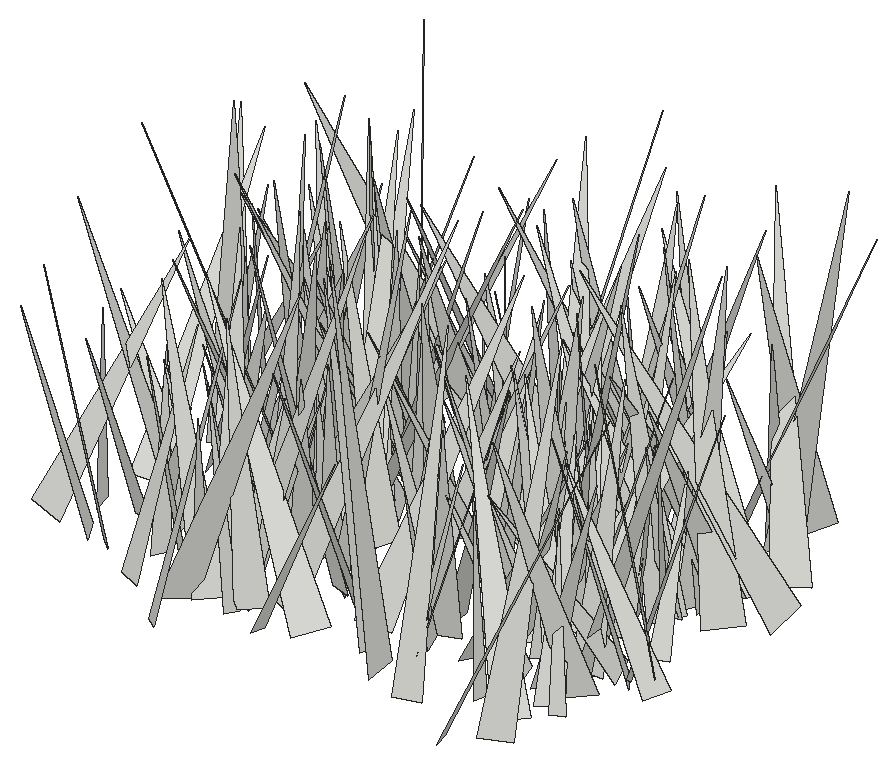
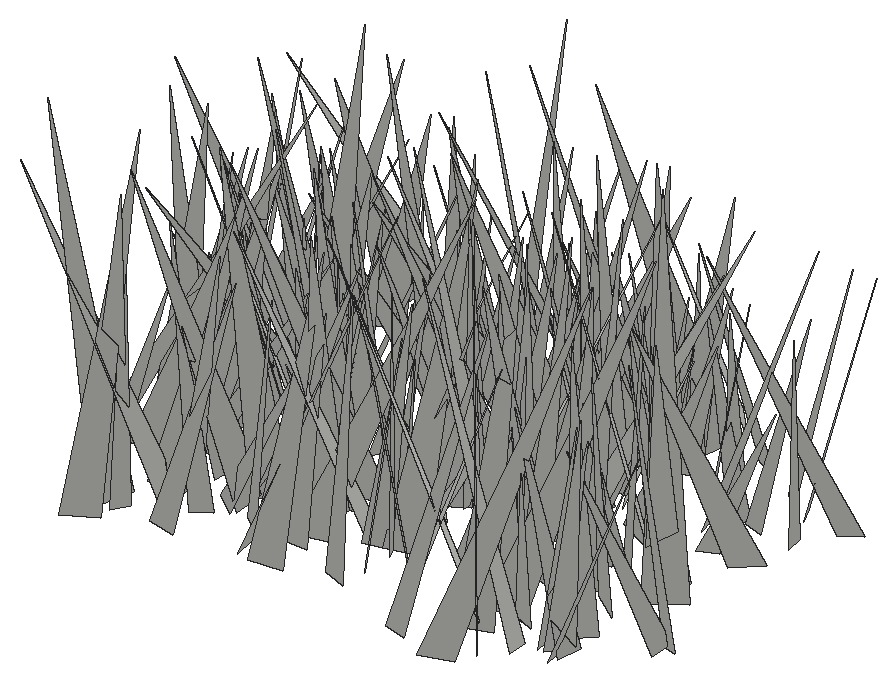
# SketchUp Ruby script. Lengths in inches.
U = 1.inch
M = Sketchup.active_model
def pt(a) = Geom::Point3d.new(a.map { |v| v * U })
def face(e, loops, mat)
  f = e.add_face(loops[0].map { |a| pt(a) })
  loops[1..].each { |l| e.add_face(l.map { |a| pt(a) }).erase! }
  f.material = f.back_material = mat if mat
  f
end
# faces: each face lists its corners as indices into pts; further lists are holes
def faces(e, pts, list, mat = nil) = list.each { |f| face(e, (f[0].is_a?(Array) ? f : [f]).map { |l| l.map { |i| pts[i] } }, mat) }
# xy, xz, yz: faces in a plane at the given z, y or x. An outline is a flat list of corners, or four numbers for a rectangle; further outlines are holes
def ring(l) = l.size == 4 ? [[l[0], l[1]], [l[2], l[1]], [l[2], l[3]], [l[0], l[3]]] : l.each_slice(2).to_a
def flat(e, list, mat, &to3) = list.each { |f| face(e, (f[0].is_a?(Array) ? f : [f]).map { |l| ring(l).map { |u, v| to3.(u, v) } }, mat) }
def xy(e, z, list, mat = nil) = flat(e, list, mat) { |x, y| [x, y, z] }
def xz(e, y, list, mat = nil) = flat(e, list, mat) { |x, z| [x, y, z] }
def yz(e, x, list, mat = nil) = flat(e, list, mat) { |y, z| [x, y, z] }
def lines(e, pts, list) = list.each { |a, b| e.add_line(pt(pts[a]), pt(pts[b])) }
# prism: a flat outline (further loops are holes) pulled along v
def prism(e, loops, v, mat = nil)
  f = face(e, loops, mat); d = Geom::Vector3d.new(v.map { |x| x * U })
  f.pushpull(f.normal.samedirection?(d) ? d.length : -d.length)
end
def box(e, o, s, mat = nil) = prism(e, [[o, [o[0] + s[0], o[1], o[2]], [o[0] + s[0], o[1] + s[1], o[2]], [o[0], o[1] + s[1], o[2]]]], [0, 0, s[2]], mat)
def at(x, y, z, deg = 0) = Geom::Transformation.translation(pt([x, y, z])) * Geom::Transformation.rotation(ORIGIN, Z_AXIS, deg.degrees)
def axes(o, x, y, z) = Geom::Transformation.new([*x, 0, *y, 0, *z, 0, *pt(o).to_a, 1])
def part(name) = M.definitions.add(name)
# library, detail: a bought-in or finely detailed component or shape, given as its bounding box
def library(name, o, s) = part(name).tap { |d| box(d.entities, o, s) }
def detail(e, o, s) = box(e.add_group.entities, o, s)
def put(e, d, t, mat = nil) = e.add_instance(d, t).tap { |i| i.material = mat if mat }
def group(e, t, mat = nil) = e.add_group.tap { |g| g.transformation = t; g.material = mat if mat }.entities
root = M.entities
c1 = part("fur_instance\#9")
p = [[0.8125,0,1.79],[0.67,-0.02,1.48],[0,-0.11,0],[0,0.11,0]]
faces(c1.entities,p,[[0,1,2,3]])
put(root,c1,axes([510.96,39.78,-21.86],[6.76451,-3.26106,1.25254],[-3.47694,-6.54929,1.72622],[-0.33809,2.1058,7.30844]))
put(root,c1,axes([520.17,40.19,-21.86],[-7.87878,-1.52664,2.20407],[-1.70967,8.13085,-0.47967],[2.06533,0.90687,8.01097]))
put(root,c1,axes([525.16,37.5,-21.86],[6.18332,3.30926,0.01495],[3.17233,-5.93637,1.96995],[-0.9422,1.73008,6.73082]))
put(root,c1,axes([514.76,39.76,-21.86],[3.9235,0.14114,0.37721],[0.06723,-3.8717,0.74932],[-0.3971,0.73898,3.85386]))
put(root,c1,axes([511.38,37.72,-21.86],[4.35483,5.04158,0.80125],[4.65214,-4.35304,2.10539],[-2.1017,0.81089,6.32055]))
put(root,c1,axes([510.83,41.33,-21.86],[3.85883,-1.0172,1.02296],[-0.87371,-3.97244,-0.65425],[-1.14794,-0.39587,3.93665]))
put(root,c1,axes([505.32,41.69,-21.86],[-4.38014,-2.49103,0.91186],[-2.44951,4.47381,0.4553],[1.01814,0.04674,5.01832]))
put(root,c1,axes([521.75,39.64,-21.86],[2.50571,3.8301,0.73521],[3.84486,-2.57244,0.29737],[-0.65369,-0.44905,4.56726]))
put(root,c1,axes([513.61,40.83,-21.86],[-3.51075,4.42455,2.16586],[4.8357,3.60279,0.47842],[0.94002,-2.00904,5.62789]))
put(root,c1,axes([511.89,40.51,-21.86],[-3.34146,5.15286,1.47209],[5.35695,3.16362,1.08579],[-0.14849,-1.82317,6.0447]))
put(root,c1,axes([508.66,39.8,-21.86],[2.03381,4.83721,0.83738],[4.90479,-2.04045,-0.1258],[-0.20703,-0.82108,5.24587]))
put(root,c1,axes([513.19,40.18,-21.86],[-4.31173,0.11749,0.33288],[0.02447,4.16916,-1.1546],[0.35215,1.14887,4.15592]))
put(root,c1,axes([506.32,41.36,-21.86],[-4.01169,-3.78695,1.3287],[-4.00574,3.89344,-0.9976],[0.2459,1.64323,5.42581]))
put(root,c1,axes([517.29,42.8,-21.86],[-2.82637,-5.01502,0.69558],[-5.06125,2.81969,-0.23605],[0.13409,0.7222,5.75179]))
put(root,c1,axes([524.34,40.86,-21.86],[-3.8319,-0.08961,1.0116],[-0.27638,3.8917,-0.7022],[0.97723,0.7493,3.76807]))
put(root,c1,axes([526.22,40.31,-21.86],[-3.78417,5.30239,0.2634],[5.25954,3.70033,1.07214],[-0.72248,-0.83479,6.42541]))
put(root,c1,axes([516.39,40.84,-21.86],[-4.44973,5.42889,0.1833],[5.21151,4.19987,2.12315],[-1.53186,-1.48148,6.69068]))
put(root,c1,axes([527.11,43.31,-21.86],[2.07945,-5.56592,1.40736],[-5.43571,-2.39045,-1.42237],[-1.84751,0.76846,5.76892]))
put(root,c1,axes([522.29,39.06,-21.86],[0.51601,7.02264,0.2402],[6.84431,-0.55684,1.57697],[-1.5908,-0.11784,6.86272]))
put(root,c1,axes([512.39,41.36,-21.86],[0.83525,-3.69964,2.10924],[-4.22949,-0.46947,0.8514],[0.49764,2.21949,3.69595]))
put(root,c1,axes([510.875,42.09,-21.86],[-2.76713,3.18046,1.2921],[3.43249,2.58898,0.97827],[0.05304,-1.61979,4.10065]))
put(root,c1,axes([526.72,38.75,-21.86],[-6.77077,3.15469,0.89527],[2.64884,6.47215,-2.77341],[1.93319,2.18084,6.93567]))
put(root,c1,axes([509.32,42.14,-21.86],[-3.57369,-1.9669,1.0397],[-2.0892,3.64317,-0.28897],[0.76478,0.76131,4.06896]))
put(root,c1,axes([520.37,42.99,-21.86],[-3.2792,-1.26365,1.37089],[-0.97388,3.52607,0.9207],[1.58988,-0.44645,3.3915]))
put(root,c1,axes([520.41,43.7,-21.86],[2.49567,-4.97649,0.70111],[-5.02561,-2.47346,0.33254],[-0.01412,0.77585,5.55727]))
put(root,c1,axes([512.63,41.28,-21.86],[4.03025,7.20792,1.49357],[7.34455,-3.82368,-1.36555],[0.49235,-1.96292,8.14446]))
put(root,c1,axes([518.88,41.26,-21.86],[-7.00273,-0.39667,0.95685],[-0.59042,6.90153,-1.45992],[0.85107,1.52402,6.86034]))
put(root,c1,axes([508.4,42.01,-21.86],[-3.76859,1.24193,1.36163],[1.17189,4.00702,-0.41131],[1.42236,-0.01087,3.94658]))
put(root,c1,axes([506.92,43.63,-21.86],[1.3305,-3.93215,0.09517],[-3.71952,-1.22514,1.38031],[1.27907,0.52755,3.91494]))
put(root,c1,axes([527.36,41.6,-21.86],[-0.19051,3.61425,0.52762],[3.57644,0.0773,0.76192],[-0.74175,-0.55561,3.53816]))
put(root,c1,axes([524.51,43.36,-21.86],[-4.25232,-1.15186,0.17503],[-1.13335,4.24309,0.38907],[0.27009,-0.33025,4.38835]))
put(root,c1,axes([506.2,43.72,-21.86],[-1.28236,-4.10189,0.60594],[-4.14572,1.27987,-0.10961],[0.07509,0.61118,4.29626]))
put(root,c1,axes([525.61,43.07,-21.86],[4.86131,-2.02952,0.59697],[-2.06386,-4.87843,0.22145],[-0.46454,0.43544,5.26329]))
put(root,c1,axes([511.71,41.88,-21.86],[-2.53684,6.34204,1.9532],[6.60869,2.60398,0.12835],[0.60133,-1.86275,6.82939]))
put(root,c1,axes([512.5,42.08,-21.86],[3.86814,-0.78573,1.02615],[-1.07279,-3.75781,1.16655],[-0.72076,1.37634,3.77081]))
put(root,c1,axes([527.2,45.56,-21.86],[-5.02387,-1.18033,0.42976],[-0.88594,4.58548,2.23734],[0.8905,-2.09699,4.65046]))
put(root,c1,axes([520.73,41.56,-21.86],[4.75922,3.00167,0.77273],[2.8511,-4.79497,1.06623],[-1.21588,0.50555,5.5248]))
put(root,c1,axes([520.0625,44.61,-21.86],[6.9866,-0.46387,0.39437],[-0.38095,-6.874,-1.33651],[-0.47495,-1.31005,6.87325]))
put(root,c1,axes([503.09,41.875,-21.86],[0.65701,6.39206,0.99008],[6.12037,-0.29236,-2.17392],[2.09278,-1.15171,6.04683]))
put(root,c1,axes([526.6875,41.98,-21.86],[-3.96377,3.38106,0.80717],[3.27975,4.04327,-0.83051],[1.15166,0.12228,5.14327]))
put(root,c1,axes([512.84,44.89,-21.86],[2.81621,-4.35059,0.38195],[-4.36621,-2.81499,0.12899],[-0.09891,0.39082,5.18093]))
put(root,c1,axes([504.32,43.65,-21.86],[3.8396,0.83392,1.68617],[0.96833,-4.16197,-0.14664],[-1.61273,-0.51356,3.92638]))
put(root,c1,axes([515.26,43.97,-21.86],[-3.81075,-5.76969,1.72606],[-6.01138,3.52106,-1.50194],[-0.36316,2.25903,6.74947]))
put(root,c1,axes([507.78,44.27,-21.86],[-6.60705,-1.5953,0.55499],[-1.61141,6.62494,-0.14037],[0.50631,0.26714,6.79547]))
put(root,c1,axes([527.81,45.21,-21.86],[-4.16981,-3.31895,0.85743],[-3.36405,4.22145,-0.01946],[0.65859,0.54939,5.32938]))
put(root,c1,axes([514.6,41.54,-21.86],[3.274,7.7332,0.0389],[7.72076,-3.26624,-0.49451],[0.44025,-0.22856,8.38313]))
put(root,c1,axes([522.1,42.8,-21.86],[4.92859,0.75105,0.39032],[0.57555,-4.66461,1.7081],[-0.62062,1.63853,4.68375]))
put(root,c1,axes([522.9,45.05,-21.86],[4.88822,-0.89007,0.63341],[-0.87396,-4.92864,-0.18113],[-0.65546,-0.06625,4.96529]))
put(root,c1,axes([529.28,45.05,-21.86],[-3.88127,2.88585,0.74535],[2.95869,3.58243,1.53633],[-0.36036,-1.66913,4.58608]))
put(root,c1,axes([509.16,45.22,-21.86],[-3.35519,-0.75879,1.11745],[-0.66434,3.53232,0.40387],[1.17606,-0.1694,3.41613]))
put(root,c1,axes([514.92,44.31,-21.86],[4.94057,6.27292,2.28459],[6.62263,-4.9638,-0.69253],[-0.84236,-2.23369,7.95482]))
put(root,c1,axes([513.32,45.86,-21.86],[4.3252,-1.84495,1.08949],[-1.74272,-4.45705,-0.62914],[-1.2465,-0.1704,4.65998]))
put(root,c1,axes([511.8,44.61,-21.86],[-1.17344,-6.36654,3.3674],[-7.15717,1.41187,0.17527],[0.80444,3.27459,6.4714]))
put(root,c1,axes([525.7,43.97,-21.86],[-3.54308,4.52564,0.44169],[4.5332,3.47169,0.79207],[-0.35583,-0.83417,5.69276]))
put(root,c1,axes([511.24,44.96,-21.86],[-3.56795,-1.90054,0.20659],[-1.88749,3.43261,-1.0196],[-0.30353,0.99505,3.91187]))
put(root,c1,axes([513.1,45.89,-21.86],[3.12862,-2.29976,0.97047],[-2.27,-3.26853,-0.42753],[-1.03819,0.21622,3.85932]))
put(root,c1,axes([511.64,46.0625,-21.86],[-2.97,-5.19915,0.68344],[-5.09037,2.66981,-1.8109],[-1.25951,1.46972,5.70725]))
put(root,c1,axes([526.1875,44.8,-21.86],[-0.55684,5.82392,2.02647],[6.12632,0.75415,-0.48394],[0.70204,-1.96161,5.83043]))
put(root,c1,axes([518.55,45.63,-21.86],[-4.66446,-0.17714,0.77084],[-0.14932,4.72517,0.1823],[0.77671,-0.15541,4.66426]))
put(root,c1,axes([527.94,46.54,-21.86],[4.20893,3.73459,3.7879],[4.59902,-4.98198,-0.19834],[-2.67289,-2.69131,5.62342]))
put(root,c1,axes([523.57,47.62,-21.86],[4.41778,-6.32124,1.65754],[-6.32459,-4.6393,-0.83587],[-1.6447,0.86086,7.66656]))
put(root,c1,axes([516.64,46.67,-21.86],[3.18493,-3.37138,0.77047],[-3.44968,-3.17103,0.3845],[-0.24394,0.82581,4.62191]))
put(root,c1,axes([524.18,44.6,-21.86],[-4.57761,1.25738,1.06742],[0.91701,4.55759,-1.43608],[1.37093,1.14988,4.52473]))
put(root,c1,axes([523.14,45.9,-21.86],[1.65832,3.59632,1.35209],[3.82471,-1.68517,-0.20869],[-0.36513,-1.31848,3.95475]))
put(root,c1,axes([517.89,42.61,-21.86],[-5.17652,4.83446,1.05401],[3.91261,4.93311,-3.41105],[3.02894,1.88989,6.20751]))
put(root,c1,axes([506.45,46.07,-21.86],[-3.16167,2.60611,0.16715],[2.5519,3.02748,1.0668],[-0.55458,-0.92652,3.956]))
put(root,c1,axes([510.97,48.55,-21.86],[7.2919,-1.58164,0.56037],[-1.39543,-7.10365,-1.89164],[-0.93186,-1.73896,7.21769]))
put(root,c1,axes([522.01,46.38,-21.86],[-5.05494,-2.22544,0.30278],[-2.23904,4.935,-1.10864],[-0.17591,1.1357,5.41072]))
put(root,c1,axes([519.49,48.05,-21.86],[-5.15654,-2.89646,0.02201],[-2.88562,5.14083,0.47427],[0.2514,-0.40276,5.89529]))
put(root,c1,axes([523.26,45.3,-21.86],[-1.86481,4.13252,0.34952],[4.14724,1.85655,0.17621],[-0.01744,-0.39104,4.53037]))
put(root,c1,axes([522.76,47.14,-21.86],[4.45339,-2.56263,0.11815],[-2.55046,-4.39735,0.75645],[0.27609,0.71411,5.08208]))
put(root,c1,axes([511.48,47,-21.86],[-6.03257,-5.76703,0.56772],[-5.59645,5.58532,-2.7307],[-1.50355,2.34912,7.8863]))
put(root,c1,axes([520.56,48,-21.86],[-4.47409,-0.55232,0.95951],[-0.288,4.43762,1.21151],[1.069,-1.11608,4.34221]))
put(root,c1,axes([511.49,46.49,-21.86],[5.54301,-4.89223,1.08245],[-4.92161,-5.01325,2.54471],[0.93987,2.60075,6.94141]))
put(root,c1,axes([524.07,48.05,-21.86],[-2.90046,-3.39812,1.38689],[-3.27993,3.19309,0.96417],[1.64705,0.37459,4.36237]))
put(root,c1,axes([525.37,46.15,-21.86],[-4.45117,0.87592,1.04433],[0.68712,4.52233,-0.86441],[1.17717,0.67238,4.45342]))
put(root,c1,axes([509.32,46.76,-21.86],[-0.49335,5.1966,1.87912],[5.02115,-0.36617,2.33091],[-2.30734,-1.90798,4.67065]))
put(root,c1,axes([526.37,44.42,-21.86],[7.79418,1.63756,2.08164],[0.8535,-7.67768,2.8441],[-2.50726,2.47704,7.43922]))
put(root,c1,axes([515.92,49.31,-21.86],[4.30968,-5.09044,0.61484],[-5.06109,-4.35201,-0.55619],[-0.82219,0.10671,6.64655]))
put(root,c1,axes([505.57,48.74,-21.86],[6.27835,0.76334,0.54412],[0.88551,-6.03847,-1.74618],[-0.30762,-1.80294,6.07875]))
put(root,c1,axes([508.95,49.41,-21.86],[-0.2881,-6.79413,1.19024],[-6.52945,0.65262,2.14482],[2.22333,1.03623,6.45314]))
put(root,c1,axes([522.2,48.43,-21.86],[-3.55733,-3.55392,1.20149],[-3.66341,3.64755,-0.05732],[0.80828,0.89081,5.02808]))
put(root,c1,axes([506.3,48.76,-21.86],[1.4923,-4.43759,0.64343],[-4.35505,-1.27294,1.3215],[1.06759,1.01025,4.49142]))
put(root,c1,axes([510.25,47.36,-21.86],[3.92442,2.27765,0.90763],[2.32456,-4.0011,-0.01041],[-0.77966,-0.46478,4.53747]))
put(root,c1,axes([521.35,48.45,-21.86],[1.81609,-4.28388,1.69446],[-4.45246,-2.09973,-0.53642],[-1.18256,1.32684,4.62191]))
put(root,c1,axes([523.42,46.4,-21.86],[7.46967,2.68884,2.29218],[2.3982,-7.79505,1.32883],[-2.59473,0.53597,7.82688]))
put(root,c1,axes([517,47.37,-21.86],[0.90877,4.85728,1.17196],[4.86719,-0.59112,-1.32422],[1.13009,-1.36012,4.76083]))
put(root,c1,axes([514.39,47.65,-21.86],[-5.92125,2.00992,1.02968],[2.02644,6.00419,-0.06686],[0.99676,-0.26678,6.25272]))
put(root,c1,axes([527.68,47.16,-21.86],[-2.23531,2.8422,0.49749],[2.78374,2.28983,-0.57415],[0.75919,-0.0278,3.57002]))
put(root,c1,axes([527.78,45.28,-21.86],[4.27823,3.00126,0.70858],[2.21616,-3.83495,2.86263],[-2.14435,2.02448,4.3722]))
put(root,c1,axes([523.77,47.72,-21.86],[5.13146,2.31605,0.71954],[2.33013,-5.17519,0.0403],[-0.67253,-0.25897,5.62978]))
put(root,c1,axes([513.23,50.17,-21.86],[-6.73685,-3.71008,0.0403],[-3.70619,6.73292,0.28887],[0.17463,-0.23362,7.68547]))
put(root,c1,axes([515.41,48.4375,-21.86],[5.69837,-0.41307,2.53776],[-0.52377,-6.22748,0.16244],[-2.51724,0.36068,5.71101]))
put(root,c1,axes([525.07,49.12,-21.86],[4.02483,1.17033,1.17041],[1.40502,-4.04247,-0.78939],[-0.87491,-1.10794,4.11653]))
put(root,c1,axes([526.42,49.07,-21.86],[-3.74193,-1.93414,1.83822],[-1.95383,4.14237,0.38123],[1.81727,0.47108,4.19495]))
put(root,c1,axes([523.44,48.6,-21.86],[1.02394,3.35387,1.44831],[3.57422,-1.23084,0.32333],[-0.75567,-1.27715,3.49176]))
put(root,c1,axes([504.61,46.04,-21.86],[-2.48989,6.58556,0.19317],[6.42005,2.47161,-1.51018],[1.47984,0.3578,6.87667]))
put(root,c1,axes([505.21,50.11,-21.86],[4.71718,-6.41333,2.08506],[-6.64537,-4.85367,0.10513],[-1.14777,1.74389,7.96063]))
put(root,c1,axes([505.85,49.8,-21.86],[4.65785,-0.69082,1.21899],[-0.53967,-4.78978,-0.65231],[-1.29303,-0.48941,4.6634]))
put(root,c1,axes([526.02,49.71,-21.86],[4.51203,-4.20905,2.90182],[-4.30887,-5.21386,-0.8628],[-2.75143,1.26279,6.10984]))
put(root,c1,axes([511.4,49.97,-21.86],[-4.57691,0.82768,1.57562],[1.18388,4.66198,0.99001],[1.32893,-1.30255,4.54457]))
put(root,c1,axes([507.61,49.41,-21.86],[-3.42106,-4.15596,2.05732],[-4.44833,3.66341,0.00339],[1.31032,1.58608,5.3829]))
put(root,c1,axes([526,49.99,-21.86],[0.76269,-3.95415,0.89534],[-4.04548,-0.80213,-0.09639],[-0.26648,0.86018,4.02588]))
put(root,c1,axes([506.65,50.34,-21.86],[5.46808,5.3055,1.78388],[5.41419,-4.38056,-3.56761],[1.42026,-3.72732,6.73205]))
put(root,c1,axes([508.35,47.15,-21.86],[-5.10797,-4.03263,5.02727],[-5.71036,5.80586,-1.14484],[2.98787,4.202,6.40647]))
put(root,c1,axes([518.97,49,-21.86],[3.29579,4.51514,1.8086],[4.80118,-3.36974,-0.33663],[-0.7786,-1.66678,5.57991]))
put(root,c1,axes([507.95,51.28,-21.86],[6.82649,-0.20783,2.36031],[0.47416,-6.93274,-1.9818],[-2.32152,-2.02711,6.5358]))
put(root,c1,axes([521.5625,48.67,-21.86],[-4.01098,-1.65554,1.8183],[-2.11594,4.09606,-0.93811],[1.25294,1.61753,4.23659]))
put(root,c1,axes([509.3,50.36,-21.86],[4.37094,-3.26497,1.75227],[-3.26747,-4.6741,-0.55863],[-1.74761,0.57306,5.42707]))
put(root,c1,axes([511.24,51.85,-21.86],[1.9027,-5.40071,0.1352],[-5.35593,-1.9045,-0.70218],[-0.70705,-0.10684,5.68285]))
put(root,c1,axes([526.97,52.2,-21.86],[3.41213,-4.67618,0.33772],[-4.46229,-3.36731,-1.54031],[-1.43828,-0.64649,5.58003]))
put(root,c1,axes([521.77,50.87,-21.86],[4.8829,2.83209,2.83107],[3.60518,-5.05239,-1.16384],[-1.7431,-2.51617,5.52349]))
put(root,c1,axes([511.64,52.32,-21.86],[-3.6044,-3.37024,0.34721],[-3.01204,3.4196,1.92476],[1.55135,-1.19103,4.54373]))
put(root,c1,axes([512.69,48.81,-21.86],[7.61599,0.93725,0.32253],[0.89381,-7.57423,0.90437],[-0.42844,0.85927,7.61996]))
put(root,c1,axes([523.25,47.08,-21.86],[-1.51427,6.54379,0.36236],[5.84338,1.51647,-2.96661],[2.96773,0.35306,6.02606]))
put(root,c1,axes([525.4375,47.625,-21.86],[1.19903,6.87384,0.5978],[6.78552,-1.2847,1.16229],[-1.25048,-0.38022,6.88014]))
put(root,c1,axes([513.64,46.93,-21.86],[-6.67493,4.02137,0.12146],[3.83511,6.43107,-2.16198],[1.21576,1.79188,7.48679]))
put(root,c1,axes([519.58,50.82,-21.86],[3.13574,-5.33007,1.5739],[-5.55752,-3.01682,0.85589],[-0.02918,1.79133,6.12454]))
put(root,c1,axes([510.38,51.5,-21.86],[-1.31696,-6.51866,1.83434],[-6.75362,1.40125,0.13086],[0.49623,1.77078,6.64907]))
put(root,c1,axes([529.42,52.43,-21.86],[-8.16776,0.06376,0.0825],[0.08376,7.86119,2.21763],[0.06209,-2.2183,7.8612]))
put(root,c1,axes([522.94,48.71,-21.86],[-2.1836,4.82414,0.14178],[4.82373,2.17653,0.23433],[-0.15514,-0.2257,5.29014]))
put(root,c1,axes([515.73,50.81,-21.86],[-2.7685,-2.84273,0.0732],[-2.6967,2.59213,-1.32656],[-0.90237,0.97511,3.73978]))
put(root,c1,axes([515.14,53.06,-21.86],[2.89826,-6.60565,0.55734],[-6.55377,-2.94663,-0.84295],[-0.99662,0.16719,7.16407]))
put(root,c1,axes([517.23,51.16,-21.86],[4.42222,0.57042,2.59632],[0.96066,-5.04183,-0.52855],[-2.47858,-0.93641,4.42741]))
put(root,c1,axes([511.15,52.28,-21.86],[8.07507,1.50255,0.4439],[1.56674,-7.73574,-2.31627],[0.00564,-2.35841,7.88031]))
put(root,c1,axes([515.67,49.9375,-21.86],[4.56915,3.9518,0.34933],[3.96081,-4.51383,-0.74378],[0.22516,-0.79028,5.99505]))
put(root,c1,axes([528.02,50.53,-21.86],[-4.89648,5.17695,2.06152],[5.4889,4.95404,0.59637],[0.96057,-1.91907,7.10075]))
put(root,c1,axes([517.16,49.66,-21.86],[-0.69382,4.82103,0.91338],[4.82167,0.84094,-0.77604],[0.90996,-0.78004,4.80848]))
put(root,c1,axes([506.09,49.13,-21.86],[-5.08982,4.44528,0.70369],[4.40622,5.13821,-0.58816],[0.91699,-0.01575,6.73207]))
put(root,c1,axes([524.67,54.5,-21.86],[4.86562,-4.5964,0.06859],[-4.19123,-4.47675,-2.68294],[-1.88818,-1.90726,6.13213]))
put(root,c1,axes([516.52,51.73,-21.86],[-4.64353,0.24048,0.81476],[0.40253,4.60984,0.93348],[0.74809,-0.98772,4.55508]))
put(root,c1,axes([509.41,54.38,-21.86],[2.70234,-6.75975,0.1599],[-6.39067,-2.60962,-2.31767],[-2.20886,-0.71979,6.90111]))
put(root,c1,axes([513.23,48.71,-21.86],[-7.30125,2.0292,0.54339],[1.84392,7.1322,-1.85816],[1.00641,1.65384,7.34664]))
put(root,c1,axes([518.67,51.84,-21.86],[3.82304,5.79974,2.60132],[6.29108,-3.01834,-2.51622],[0.9089,-3.50316,6.47466]))
put(root,c1,axes([525.52,51.81,-21.86],[-5.14523,1.96025,0.06602],[1.88898,4.90265,1.64806],[-0.52792,-1.56261,5.25356]))
put(root,c1,axes([526.19,51.08,-21.86],[6.73151,-1.98165,2.55494],[-2.23492,-7.11595,0.36912],[-2.33662,1.09735,7.00742]))
put(root,c1,axes([511.2,51.96,-21.86],[5.28351,-1.61661,1.62366],[-1.56193,-5.52709,-0.42043],[-1.67632,0.05465,5.50927]))
put(root,c1,axes([513.01,52.24,-21.86],[-0.75955,-3.70224,0.74684],[-3.72635,0.61048,-0.76351],[-0.61539,0.87293,3.70143]))
put(root,c1,axes([517.11,50.53,-21.86],[-3.90269,-1.36809,1.23152],[-1.73858,3.68797,-1.41263],[0.60468,1.77384,3.88679]))
put(root,c1,axes([511.14,51.32,-21.86],[4.24793,5.0228,3.04998],[5.34423,-4.86703,0.57187],[-2.44337,-1.91294,6.55335]))
put(root,c1,axes([512.5,48.67,-21.86],[-0.64935,7.68845,0.01437],[7.6155,0.6412,1.06165],[-1.05669,-0.10353,7.64243]))
put(root,c1,axes([526.55,51.27,-21.86],[-6.69372,-1.63538,1.73187],[-1.91789,6.76382,-1.02573],[1.41263,1.43387,6.81383]))
put(root,c1,axes([518.58,54.37,-21.86],[-6.66712,2.68909,2.42043],[3.53397,5.92752,3.14894],[0.77508,-3.89533,6.46266]))
put(root,c1,axes([522.32,49.48,-21.86],[5.47327,5.90798,0.9862],[5.7796,-5.55993,1.23167],[-1.57262,0.12835,7.95889]))
put(root,c1,axes([502.96,52.71,-21.86],[-1.89095,-4.65132,2.366],[-4.60338,2.67208,1.57395],[2.45798,1.42605,4.76793]))
put(root,c1,axes([520.46,51.88,-21.86],[4.16572,3.95636,0.93283],[4.06431,-4.03236,-1.04767],[0.06588,-1.40123,5.64875]))
put(root,c1,axes([512.21,51.72,-21.86],[1.76175,3.91399,1.38102],[4.01071,-1.99148,0.5277],[-1.06803,-1.02224,4.25965]))
put(root,c1,axes([506.03,53.93,-21.86],[4.00821,-3.73033,0.31245],[-3.73197,-4.01777,-0.09299],[-0.29215,0.14465,5.47471]))
put(root,c1,axes([516.2,53.34,-21.86],[1.70929,-4.46495,1.67991],[-4.63149,-1.98085,-0.55231],[-1.1433,1.34907,4.74893]))
put(root,c1,axes([525.01,54.86,-21.86],[-0.03159,-6.8611,0.78211],[-6.88005,-0.03586,-0.59249],[-0.59273,0.78192,6.83555]))
put(root,c1,axes([506.82,51.63,-21.86],[2.34142,5.16985,1.64131],[5.10687,-2.70355,1.23051],[-1.82787,-0.93109,5.54034]))
put(root,c1,axes([518.4,50.6875,-21.86],[0.38295,8.08113,1.09098],[7.9956,-0.1576,-1.6392],[1.60161,-1.14545,7.92239]))
put(root,c1,axes([515.57,53.21,-21.86],[-4.21315,-2.34987,2.26772],[-2.4638,4.71684,0.31027],[2.14339,0.80291,4.81418]))
put(root,c1,axes([521.89,52.46,-21.86],[-6.207,1.9177,0.03314],[1.91765,6.20287,0.22937],[-0.03607,-0.22893,6.49244]))
put(root,c1,axes([509.59,55.96,-21.86],[2.10072,-7.09935,0.00934],[-7.09522,-2.09917,0.25546],[0.24231,0.08144,7.39923]))
put(root,c1,axes([521.48,52.9,-21.86],[3.63637,-5.76719,3.12725],[-6.51934,-3.57646,0.98508],[-0.73369,3.19558,6.74635]))
put(root,c1,axes([503.17,52.86,-21.86],[4.26787,-0.90452,0.30078],[-0.95208,-4.11231,1.14272],[-0.04649,1.18073,4.21035]))
put(root,c1,axes([522.52,54.37,-21.86],[-2.43952,-3.83837,0.4143],[-3.75379,2.24378,-1.31547],[-0.90209,1.04325,4.3536]))
put(root,c1,axes([515.53,54.86,-21.86],[-3.34648,-2.86729,1.25208],[-2.75468,3.56945,0.81158],[1.4835,0.16004,4.33146]))
put(root,c1,axes([527.3125,52.86,-21.86],[-3.78872,6.01371,0.63065],[5.87535,3.48538,2.06137],[-1.42923,-1.61377,6.8022]))
put(root,c1,axes([523.95,52.54,-21.86],[-3.54385,2.2292,0.7922],[1.93522,3.55225,-1.33876],[1.36083,0.75365,3.96686]))
put(root,c1,axes([519.18,52.57,-21.86],[-5.31707,5.30249,0.96243],[5.27581,5.39738,-0.58989],[1.09932,-0.2564,7.48596]))
put(root,c1,axes([519.72,56.7,-21.66],[-6.83596,-2.73328,0.53057],[-2.58478,6.75268,1.48423],[1.035,-1.18879,7.21098]))
put(root,c1,axes([522.63,55.63,-21.66],[0.54307,-5.39112,1.14857],[-5.29865,-0.1925,1.60174],[1.51911,1.25582,5.17624]))
put(root,c1,axes([505.91,55.91,-21.86],[-4.07009,-1.55263,0.42821],[-1.43545,4.0247,0.94922],[0.73043,-0.7422,4.25151]))
put(root,c1,axes([506.82,54.65,-21.86],[-3.50037,2.65675,1.28484],[2.86731,3.53339,0.50538],[0.69832,-1.19104,4.36526]))
put(root,c1,axes([521.87,53.61,-21.86],[7.1879,-0.3196,1.18159],[-0.53762,-7.14753,1.33717],[-1.09967,1.40532,7.06966]))
put(root,c1,axes([518.7,55.11,-21.86],[0.55696,-4.64877,2.01019],[-4.98122,-0.86859,-0.62855],[-0.91614,1.89648,4.63963]))
put(root,c1,axes([526.96,56.09,-21.86],[0.09538,-4.31944,0.7575],[-4.29634,-0.24392,-0.84995],[-0.8791,0.72346,4.23607]))
put(root,c1,axes([520.74,54.99,-21.86],[2.49829,3.83803,2.30798],[4.11646,-3.0089,0.54773],[-1.76409,-1.58579,4.54664]))
put(root,c1,axes([507.4,56.1,-21.86],[6.89965,2.05968,0.48381],[2.11498,-6.67017,-1.76557],[0.05673,-1.82978,6.98071]))
put(root,c1,axes([505.66,55.22,-21.86],[4.85484,-0.93426,0.93937],[-1.01134,-4.91828,0.33525],[-0.85583,0.51221,4.93253]))
put(root,c1,axes([508.45,54.4,-21.86],[0.5097,3.85536,0.87755],[3.83119,-0.70034,0.85159],[-0.9777,-0.73445,3.79452]))
put(root,c1,axes([506.87,55.0625,-21.86],[-5.03296,-0.41167,1.23228],[-0.52474,5.15421,-0.42127],[1.18855,0.5323,5.03216]))
put(root,c1,axes([511.69,57.91,-21.86],[-2.17037,-5.72704,0.1674],[-5.69455,2.17595,0.61228],[0.63178,-0.0613,6.09382]))
put(root,c1,axes([517.46,52.29,-21.86],[6.25178,5.32919,0.93445],[4.93149,-6.20008,2.36594],[-2.22574,1.23164,7.86685]))
put(root,c1,axes([511.93,57.5,-21.86],[-3.92471,-3.72483,0.22437],[-3.66233,3.90735,0.80501],[0.71557,-0.43166,5.35067]))
put(root,c1,axes([509.73,55.39,-21.66],[5.9079,4.20697,0.32991],[4.15488,-5.69984,-1.72033],[0.73785,-1.5887,7.04573]))
put(root,c1,axes([506.05,55.28,-21.86],[3.17127,-3.30736,3.04126],[-3.82504,-3.9403,-0.2965],[-2.35731,1.94429,4.57249]))
put(root,c1,axes([513.41,54.78,-21.86],[3.52114,3.87417,1.40413],[3.91467,-3.72163,0.45161],[-1.28689,-0.72073,5.21571]))
put(root,c1,axes([515.92,56.19,-21.86],[-1.84582,-5.09705,1.94608],[-5.40108,1.99766,0.10933],[0.77171,1.78987,5.41987]))
put(root,c1,axes([525.15,57.22,-21.66],[5.21183,-0.69159,1.00189],[-0.40075,-5.13378,-1.45906],[-1.14955,-1.3458,5.051]))
put(root,c1,axes([509.28,58.52,-21.86],[-7.12654,1.94071,2.81889],[3.04033,6.57978,3.15641],[1.57127,-3.9294,6.67765]))
put(root,c1,axes([518.53,56.99,-21.86],[1.47343,-6.07806,1.78682],[-6.21699,-1.74005,-0.79238],[-1.21846,1.52838,6.20371]))
put(root,c1,axes([523.27,57.17,-21.86],[-0.49716,-5.04462,0.80589],[-5.07325,0.39247,-0.67299],[-0.59982,0.86174,5.02418]))
put(root,c1,axes([524.24,54.39,-21.86],[-6.81045,0.95525,0.6863],[0.79996,6.71798,-1.4123],[0.86231,1.31226,6.73054]))
put(root,c1,axes([526.13,58.4,-21.86],[5.76412,-4.56343,1.38579],[-4.26746,-5.90574,-1.69745],[-2.12934,-0.51736,7.15322]))
put(root,c1,axes([528.03,54.44,-21.86],[-2.86004,7.00076,0.77945],[7.00763,2.7424,1.08181],[-0.71502,-1.12544,7.48466]))
put(root,c1,axes([524.68,55.02,-21.86],[7.12948,2.21776,0.41944],[2.17259,-7.11974,0.71624],[-0.61174,0.56098,7.43203]))
put(root,c1,axes([525.96,56.64,-21.86],[7.67247,-2.21843,2.0813],[-2.41925,-7.8734,0.52613],[-1.84403,1.09916,7.96941]))
put(root,c1,axes([508.78,56.75,-21.86],[-5.8561,-4.67693,3.47291],[-5.12361,6.47844,0.0849],[2.77191,2.09401,7.49403]))
